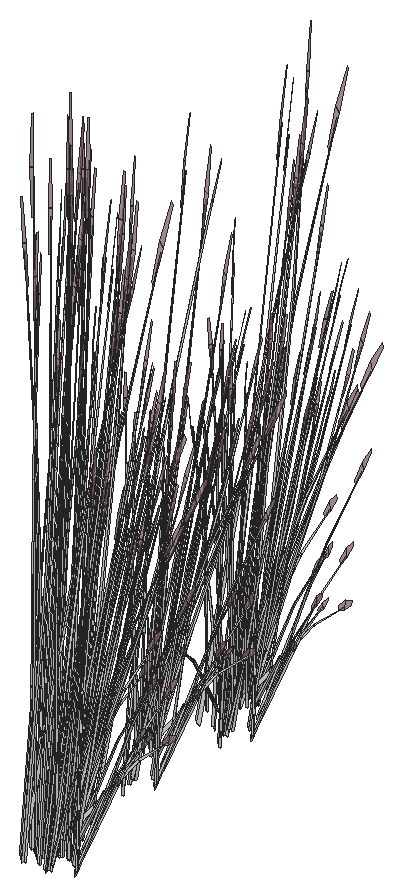
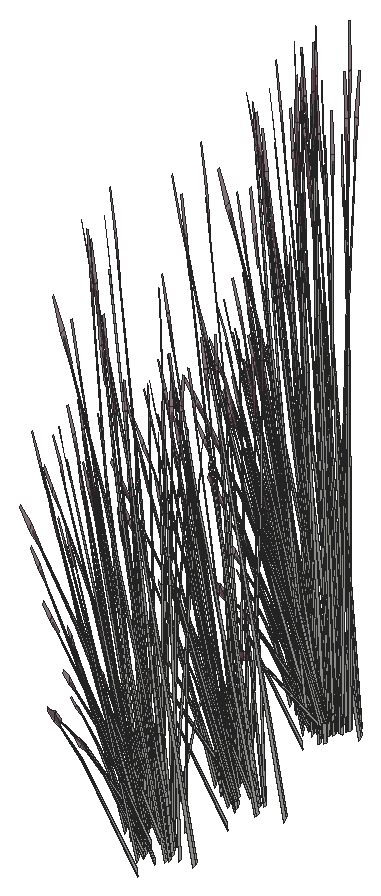
# SketchUp Ruby script. Lengths in inches.
U = 1.inch
M = Sketchup.active_model
def pt(a) = Geom::Point3d.new(a.map { |v| v * U })
def face(e, loops, mat)
  f = e.add_face(loops[0].map { |a| pt(a) })
  loops[1..].each { |l| e.add_face(l.map { |a| pt(a) }).erase! }
  f.material = f.back_material = mat if mat
  f
end
# faces: each face lists its corners as indices into pts; further lists are holes
def faces(e, pts, list, mat = nil) = list.each { |f| face(e, (f[0].is_a?(Array) ? f : [f]).map { |l| l.map { |i| pts[i] } }, mat) }
# xy, xz, yz: faces in a plane at the given z, y or x. An outline is a flat list of corners, or four numbers for a rectangle; further outlines are holes
def ring(l) = l.size == 4 ? [[l[0], l[1]], [l[2], l[1]], [l[2], l[3]], [l[0], l[3]]] : l.each_slice(2).to_a
def flat(e, list, mat, &to3) = list.each { |f| face(e, (f[0].is_a?(Array) ? f : [f]).map { |l| ring(l).map { |u, v| to3.(u, v) } }, mat) }
def xy(e, z, list, mat = nil) = flat(e, list, mat) { |x, y| [x, y, z] }
def xz(e, y, list, mat = nil) = flat(e, list, mat) { |x, z| [x, y, z] }
def yz(e, x, list, mat = nil) = flat(e, list, mat) { |y, z| [x, y, z] }
def lines(e, pts, list) = list.each { |a, b| e.add_line(pt(pts[a]), pt(pts[b])) }
# prism: a flat outline (further loops are holes) pulled along v
def prism(e, loops, v, mat = nil)
  f = face(e, loops, mat); d = Geom::Vector3d.new(v.map { |x| x * U })
  f.pushpull(f.normal.samedirection?(d) ? d.length : -d.length)
end
def box(e, o, s, mat = nil) = prism(e, [[o, [o[0] + s[0], o[1], o[2]], [o[0] + s[0], o[1] + s[1], o[2]], [o[0], o[1] + s[1], o[2]]]], [0, 0, s[2]], mat)
def at(x, y, z, deg = 0) = Geom::Transformation.translation(pt([x, y, z])) * Geom::Transformation.rotation(ORIGIN, Z_AXIS, deg.degrees)
def axes(o, x, y, z) = Geom::Transformation.new([*x, 0, *y, 0, *z, 0, *pt(o).to_a, 1])
def part(name) = M.definitions.add(name)
# library, detail: a bought-in or finely detailed component or shape, given as its bounding box
def library(name, o, s) = part(name).tap { |d| box(d.entities, o, s) }
def detail(e, o, s) = box(e.add_group.entities, o, s)
def put(e, d, t, mat = nil) = e.add_instance(d, t).tap { |i| i.material = mat if mat }
def group(e, t, mat = nil) = e.add_group.tap { |g| g.transformation = t; g.material = mat if mat }.entities
root = M.entities
M.materials.add("LightPink_Translucent").color = [144, 107, 117]
M.materials["LightPink_Translucent"].alpha = 0.75
c1 = part("blade")
p = [[2.15,0.21,22],[0,0.17,0],[0.09,0.45,0],[2.18,0.31,22],[2.29,0.31,22],[0.38,0.45,0],
  [2.48,0.24,33],[2.49,0.24,33],[2.48,0.22,33]]
faces(c1.entities,p,[[0,1,2,3],[4,5,2,3],[6,3,4,7],[8,0,3,6]])
c2 = part("seeds")
p = [[0.3,-0.1,1.38],[-0.01,-0.03,1.59],[-0.01,-0.03,0.03],[0.14,-0.07,-0.07],[0.29,-0.03,3],[0.15,0.01,3.11]]
faces(c2.entities,p,[[0,1,2,3],[1,0,4,5]],"LightPink_Translucent")
c3 = part("blade with seeds")
put(c3.entities,c1,at(0,0,0))
put(c3.entities,c2,axes([2.4,0.25,30.99],[1.5799,-0.05474,1.17369],[-0.12525,1.92788,0.29478],[-0.07173,-0.02425,1.56792]))
put(root,c3,axes([408.35,394.05,-9.42],[-0.17034,0.27669,1.06958],[-0.14642,-0.37174,0.78586],[0.14069,-0.09315,0.23558]))
put(root,c3,axes([408.1,395.09,-7.78],[0.44516,-0.07768,-0.32977],[0.11755,0.44407,0.42575],[0.12757,-0.11927,0.81462]))
put(root,c3,axes([405.49,395.5,-9.52],[-0.05959,-0.62022,-0.27094],[0.62068,-0.0375,-0.46562],[0.1093,-0.08261,1.4872]))
put(root,c3,axes([407.74,395.36,-7.3],[-0.44516,0.07768,0.32977],[-0.11755,-0.44407,-0.42575],[0.12757,-0.11927,0.81462]))
put(root,c3,axes([405.41,394.125,-10.11],[0.47712,0.13449,-0.28847],[-0.12013,0.47362,0.28847],[0.09619,-0.05462,1.29413]))
put(root,c3,axes([408.14,395.29,-7.6],[0.35109,0.22859,0.05988],[-0.2044,0.32553,0.47138],[0.11256,-0.10524,0.71878]))
put(root,c3,axes([408.05,395.1875,-7.59],[0.12683,0.50025,0.447],[-0.49754,0.08682,0.36857],[0.14663,-0.11765,0.92496]))
put(root,c3,axes([409.39,395.79,-7.61],[0.07097,-0.08279,1.62908],[-0.09083,-0.50786,-0.25764],[0.17806,-0.09629,0.13065]))
put(root,c3,axes([405.57,395.98,-9.73],[0.57623,0.26344,0.22409],[-0.27732,0.5474,0.46562],[0,-0.12618,1.49497]))
put(root,c3,axes([405.39,395.62,-9.47],[-0.55535,0.03355,0.41661],[-0.05022,-0.55698,-0.2005],[0.09942,-0.05645,1.33761]))
put(root,c3,axes([407.99,396.57,-7.3125],[-0.25732,-0.49218,-0.11324],[0.45669,-0.24187,-0.62851],[0.19245,-0.06494,0.95501]))
put(root,c3,axes([407.97,396.14,-7.64],[0.13855,-0.49442,-0.47583],[0.47502,0.16947,-0.36857],[0.19125,-0.04534,0.91046]))
put(root,c3,axes([407.22,394.13,-9.79],[0.31974,-0.54466,0],[0.53494,0.30375,-0.48057],[0.12184,0.06918,1.52448]))
put(root,c3,axes([408.48,396.28,-10.15],[-0.32938,0.06523,1.31842],[-0.05243,-0.51922,0.07547],[0.2307,-0.07859,0.75023]))
put(root,c3,axes([409.08,395.82,-9.89],[-0.31706,-0.34757,-0.06041],[0.34725,-0.31847,-0.27392],[0.09839,-0.02242,0.90349]))
put(root,c3,axes([406.17,395.87,-9.95],[0,-0.62892,0],[0.63949,0,0],[0,0,1.6711]))
put(root,c3,axes([406.94,394.41,-9.69],[-0.47863,-0.27177,0.46235],[0.28609,-0.48733,0],[0.10901,0.0619,1.46668]))
put(root,c3,axes([407.88,396.32,-7.36],[0.44939,-0.24006,-0.66157],[0.25044,0.49415,0.07984],[0.21713,-0.05613,0.93586]))
put(root,c3,axes([405.86,395.47,-9.8],[-0.42403,0.49328,0.42607],[-0.50377,-0.43543,0.16719],[0.10223,-0.04923,1.47927]))
put(root,c3,axes([405.125,394.66,-9.7],[-0.14774,0.54019,0.16428],[-0.54062,-0.15287,0.32672],[0.09339,-0.00263,1.49371]))
put(root,c3,axes([407.8125,396.42,-7.3],[-0.42502,-0.15163,0.32977],[0.12396,-0.44238,-0.42575],[0.17112,-0.04056,0.81462]))
put(root,c3,axes([404.9,395.1,-10.52],[-0.50338,0.21762,1.20058],[-0.16022,-0.62439,0.4665],[0.30911,0.01039,1.36553]))
put(root,c3,axes([406.26,395.26,-9.5625],[0.09866,-0.48509,0.13483],[0.48202,0.0842,-0.38503],[0.08772,0.04981,1.18024]))
put(root,c3,axes([408.83,395.94,-10.61],[-0.02673,-0.08252,1.6421],[0.18538,-0.48271,-0.25086],[0.187,-0.00694,0.2797]))
put(root,c3,axes([406.05,395.39,-9.47],[-0.30722,-0.45622,0.41661],[0.46535,-0.32126,-0.2005],[0.09942,0.05645,1.33761]))
put(root,c3,axes([406.21,395.42,-9.52],[0.51635,-0.36087,-0.27094],[0.34336,0.5099,-0.46562],[0.1274,0.05178,1.4872]))
put(root,c3,axes([408.26,396.37,-7.78],[0.42502,0.15163,-0.32977],[-0.12396,0.44238,0.42575],[0.17112,-0.04056,0.81462]))
put(root,c3,axes([407.51,394.46,-10.12],[0.47863,0.27177,-0.46235],[-0.28609,0.48733,0],[0.10901,0.0619,1.46668]))
put(root,c3,axes([406.6,396.01,-9.95],[0.57217,0,0],[0,0.56272,0],[0,0,1.66132]))
put(root,c3,axes([406.76,394.6875,-9.7],[-0.54955,0.14427,0.16428],[-0.1357,-0.53689,0.32672],[0.04901,0.07823,1.49371]))
put(root,c3,axes([407.1,395.82,-8.39],[-0.21212,0.01231,1.59586],[0.14072,-0.53355,0.12904],[0.3023,0.033,0.68222]))
put(root,c3,axes([407.375,394.66,-10.11],[0.12013,0.47362,-0.28847],[-0.47712,0.13449,0.28847],[0.09619,0.05462,1.29413]))
put(root,c3,axes([408.2,396.56,-7.6],[0.18783,0.37061,0.05988],[-0.34252,0.1814,0.47138],[0.15099,-0.03579,0.71878]))
put(root,c3,axes([406.42,395.72,-9.78],[-0.64638,-0.11452,0.45814],[0.13155,-0.64678,0.17978],[0.09446,0.06245,1.59061]))
put(root,c3,axes([408.16,396.42,-7.59],[-0.14449,0.4956,0.447],[-0.47502,-0.16947,0.36857],[0.1868,-0.02978,0.92496]))
put(root,c3,axes([406.52,397.25,-9.97],[0.53691,-0.18442,-0.17877],[0.18866,0.53125,0.00007],[0.05927,-0.02038,1.61933]))
put(root,c3,axes([406.59,396.25,-9.9375],[0.35699,0.35109,0],[-0.35699,0.35109,0],[0,0,1.57621]))
put(root,c3,axes([407.55,396.1,-9.7],[-0.40181,-0.39593,0.16428],[0.40492,-0.38402,0.32672],[-0.04438,0.08086,1.49371]))
put(root,c3,axes([406.81,395.5,-10.08],[0.53199,0.08911,-0.58063],[-0.11226,0.54969,-0.15239],[0.15876,0.06661,1.28164]))
put(root,c3,axes([409.16,396.46,-9.42],[-0.31598,0.08973,1.06958],[0.14873,-0.37085,0.78586],[0.16763,0.02538,0.23558]))
put(root,c3,axes([406.58,395.84,-9.47],[0.24813,-0.48978,0.41661],[0.51557,0.23571,-0.2005],[0,0.1129,1.33761]))
put(root,c3,axes([409.01,398.03,-7.62],[-0.04624,-0.04758,1.65179],[0.10116,-0.51007,-0.15608],[0.18215,-0.03259,0.29231]))
put(root,c3,axes([406.49,396.12,-9.87],[0,0.62861,-0.05249],[-0.63949,0,0],[0,0.01975,1.67027]))
put(root,c3,axes([406.53,395.67,-9.94],[0.30722,0.45622,-0.41661],[-0.46535,0.32126,0.2005],[0.09942,0.05645,1.33761]))
put(root,c3,axes([408.61,397.6,-8.34],[-0.09788,-0.45691,-0.03251],[0.46264,-0.10504,-0.14742],[0.09661,0.02897,0.48626]))
put(root,c3,axes([407.41,397.59,-7.3125],[0.02738,-0.55277,-0.11324],[0.51847,0.01511,-0.62851],[0.19968,0.0384,0.95501]))
put(root,c3,axes([407.89,396.11,-9.69],[0,-0.54355,0.46235],[0.57217,0,0],[0,0.1238,1.46668]))
put(root,c3,axes([406.8,395.95,-9.5625],[0.47648,-0.15851,0.13483],[0.16686,0.45265,-0.38503],[0,0.09962,1.18024]))
put(root,c3,axes([407.33,397.37,-7.3],[-0.29098,-0.34031,0.32977],[0.33226,-0.32215,-0.42575],[0.16881,0.04902,0.81462]))
put(root,c3,axes([408.57,397.05,-9.59],[-0.12317,-0.13368,1.33163],[0.16025,-0.44223,-0.28638],[0.24919,0.05991,0.56934]))
put(root,c3,axes([406.37,397.54,-9.95],[0.51557,0.24403,0],[-0.24813,0.50705,0],[0,0,1.62917]))
put(root,c3,axes([407.86,397.26,-7.61],[0.10971,-0.00919,1.62908],[0.30091,-0.42228,-0.25764],[0.19514,0.05574,0.13065]))
put(root,c3,axes([407.4375,397.32,-7.36],[0.51122,0.01309,-0.66157],[-0.03434,0.5511,0.07984],[0.21658,0.05816,0.93586]))
put(root,c3,axes([406.18,397.34,-9.87],[0.22235,0.62444,-0.05599],[-0.63531,0.21881,0],[0.00776,0.02181,1.60327]))
put(root,c3,axes([408.27,396.2,-9.79],[0.63949,0,0],[0,0.60749,-0.48057],[0,0.13836,1.52448]))
put(root,c3,axes([408.02,396.52,-9.95],[-0.63917,-0.00435,-0.04634],[0,-0.60749,0.46507],[-0.02009,0.13829,1.47457]))
put(root,c3,axes([406.63,395.99,-9.52],[0.57594,0.25935,-0.27094],[-0.27732,0.5474,-0.46562],[0.0181,0.1344,1.4872]))
put(root,c3,axes([407.75,397.55,-7.78],[0.29098,0.34031,-0.32977],[-0.33226,0.32215,0.42575],[0.16881,0.04902,0.81462]))
put(root,c3,axes([407.89,396.6,-10.11],[-0.35699,0.33913,-0.28847],[-0.35699,-0.33913,0.28847],[0,0.10923,1.29413]))
put(root,c3,axes([407.6,397.68,-7.6],[-0.02575,0.41332,0.05988],[-0.38885,-0.01133,0.47138],[0.14895,0.04325,0.71878]))
put(root,c3,axes([407.63,397.55,-7.59],[-0.37709,0.35815,0.447],[-0.32522,-0.38035,0.36857],[0.17692,0.06607,0.92496]))
put(root,c3,axes([406.43,397.96,-7.3],[-0.07899,-0.43781,0.32977],[0.45153,-0.11561,-0.42575],[0.12128,0.12546,0.81462]))
put(root,c3,axes([408.13,396.62,-10.12],[0,0.54355,-0.46235],[-0.57217,0,0],[0,0.1238,1.46668]))
put(root,c3,axes([406.7,396.68,-8.39],[-0.18996,-0.09365,1.59586],[0.39312,-0.39287,0.12904],[0.24502,0.17723,0.68222]))
put(root,c3,axes([406.74,395.44,-7.83],[-0.44191,-0.28242,1.28769],[0.46662,-0.43971,0.5556],[0.14258,0.26499,1.24467]))
put(root,c3,axes([407.4,397.74,-9.42],[-0.28795,-0.15629,1.06958],[0.37181,-0.1588,0.78586],[0.10029,0.13452,0.23558]))
put(root,c3,axes([406.39,398.19,-7.3125],[0.30474,-0.46525,-0.11324],[0.44133,0.26804,-0.62851],[0.15341,0.13145,0.95501]))
put(root,c3,axes([405.99,398.58,-7.62],[0.00151,-0.06581,1.65179],[0.43826,-0.29033,-0.15608],[0.15223,0.10363,0.29231]))
put(root,c3,axes([407.48,398.32,-10.61],[0.03726,-0.07847,1.6421],[0.46909,-0.23111,-0.25086],[0.14221,0.11962,0.2797]))
put(root,c3,axes([406.87,396.54,-10.05],[0.18752,0.49766,-0.6445],[-0.54017,0.17923,-0.16915],[0.02073,0.16852,1.42262]))
put(root,c3,axes([406.75,397.96,-7.64],[0.50465,-0.12921,-0.47583],[0.08828,0.48932,-0.36857],[0.13555,0.14022,0.91046]))
put(root,c3,axes([405.35,398.03,-7.3],[0.15418,-0.41799,0.32977],[0.44981,0.12192,-0.42575],[0.04124,0.16829,0.81462]))
put(root,c3,axes([407.45,398.46,-9.52],[-0.32795,-0.01705,0.97832],[0.21658,-0.36206,0.54015],[0.12956,0.12863,0.76741]))
put(root,c3,axes([406.5,398.36,-7.6],[-0.23243,0.34529,0.05988],[-0.331,-0.20103,0.47138],[0.10701,0.1107,0.71878]))
put(root,c3,axes([405.96,399.52,-6.74],[0.35341,-0.31182,-0.06041],[0.32382,0.34152,-0.27392],[0.0228,0.09677,0.90349]))
put(root,c3,axes([406.6,398.26,-7.59],[-0.50866,0.12474,0.447],[-0.08828,-0.48932,0.36857],[0.11963,0.14421,0.92496]))
put(root,c3,axes([406.38,397.58,-9.59],[0.00902,-0.18018,1.33163],[0.43127,-0.20126,-0.28638],[0.13313,0.21566,0.56934]))
put(root,c3,axes([405.2,398.21,-7.3125],[0.50045,-0.25306,-0.11324],[0.24593,0.44915,-0.62851],[0.06603,0.18927,0.95501]))
put(root,c3,axes([405.63,398.1875,-7.64],[0.50273,0.13626,-0.47583],[-0.17232,0.46717,-0.36857],[0.0461,0.18809,0.91046]))
put(root,c3,axes([405.92,397.22,-8.39],[-0.1169,-0.17452,1.59586],[0.54019,-0.14692,0.12904],[0.12209,0.27397,0.68222]))
put(root,c3,axes([405.45,398.1,-7.36],[0.24409,0.44196,-0.66157],[-0.50245,0.2463,0.07984],[0.05708,0.21354,0.93586]))
put(root,c3,axes([405.08,399.21,-7.61],[0.06483,0.08753,1.62908],[0.52315,0.03439,-0.25764],[0.05261,0.19303,0.13065]))
put(root,c3,axes([404.36,407.02,-10.61],[-0.07655,-0.04282,1.6421],[-0.19662,-0.47839,-0.25086],[0.13264,-0.12982,0.2797]))
put(root,c3,axes([404.36,408.37,-7.36],[0.26714,-0.42887,-0.66157],[0.46811,0.30479,0.07984],[0.1595,-0.15539,0.93586]))
put(root,c3,axes([404.35,408.17,-7.64],[-0.13138,-0.49631,-0.47583],[0.49754,-0.08682,-0.36857],[0.14258,-0.13331,0.91046]))
put(root,c3,axes([404.58,408.52,-7.3125],[-0.47307,-0.29971,-0.11324],[0.27254,-0.43404,-0.62851],[0.13365,-0.15087,0.95501]))
put(root,c3,axes([404.75,407.98,-9.59],[-0.1827,-0.0161,1.33163],[-0.18717,-0.43188,-0.28638],[0.22444,-0.12218,0.56934]))
put(root,c3,axes([405.75,408.39,-7.62],[-0.0668,-0.00413,1.65179],[-0.27738,-0.44233,-0.15608],[0.11139,-0.14544,0.29231]))
put(root,c3,axes([404.96,407.18,-9.42],[-0.17034,0.27669,1.06958],[-0.14642,-0.37174,0.78586],[0.14069,-0.09315,0.23558]))
put(root,c3,axes([404.71,408.22,-7.78],[0.44516,-0.07768,-0.32977],[0.11755,0.44407,0.42575],[0.12757,-0.11927,0.81462]))
put(root,c3,axes([404.75,408.41,-7.6],[0.35109,0.22859,0.05988],[-0.2044,0.32553,0.47138],[0.11256,-0.10524,0.71878]))
put(root,c3,axes([404.66,408.32,-7.59],[0.12683,0.50025,0.447],[-0.49754,0.08682,0.36857],[0.14663,-0.11765,0.92496]))
put(root,c3,axes([406,408.92,-7.61],[0.07097,-0.08279,1.62908],[-0.09083,-0.50786,-0.25764],[0.17806,-0.09629,0.13065]))
put(root,c3,axes([404.6,409.69,-7.3125],[-0.25732,-0.49218,-0.11324],[0.45669,-0.24187,-0.62851],[0.19245,-0.06494,0.95501]))
put(root,c3,axes([404.58,409.27,-7.64],[0.13855,-0.49442,-0.47583],[0.47502,0.16947,-0.36857],[0.19125,-0.04534,0.91046]))
put(root,c3,axes([403.83,407.26,-9.79],[0.31974,-0.54466,0],[0.53494,0.30375,-0.48057],[0.12184,0.06918,1.52448]))
put(root,c3,axes([405.09,409.41,-10.15],[-0.32938,0.06523,1.31842],[-0.05243,-0.51922,0.07547],[0.2307,-0.07859,0.75023]))
put(root,c3,axes([405.69,408.95,-9.89],[-0.31706,-0.34757,-0.06041],[0.34725,-0.31847,-0.27392],[0.09839,-0.02242,0.90349]))
put(root,c3,axes([404.49,409.45,-7.36],[0.44939,-0.24006,-0.66157],[0.25044,0.49415,0.07984],[0.21713,-0.05613,0.93586]))
put(root,c3,axes([404.42,409.55,-7.3],[-0.42502,-0.15163,0.32977],[0.12396,-0.44238,-0.42575],[0.17112,-0.04056,0.81462]))
put(root,c3,axes([401.51,408.22,-10.52],[-0.50338,0.21762,1.20058],[-0.16022,-0.62439,0.4665],[0.30911,0.01039,1.36553]))
put(root,c3,axes([405.44,409.07,-10.61],[-0.02673,-0.08252,1.6421],[0.18538,-0.48271,-0.25086],[0.187,-0.00694,0.2797]))
put(root,c3,axes([404.87,409.5,-7.78],[0.42502,0.15163,-0.32977],[-0.12396,0.44238,0.42575],[0.17112,-0.04056,0.81462]))
put(root,c3,axes([404.12,407.59,-10.12],[0.47863,0.27177,-0.46235],[-0.28609,0.48733,0],[0.10901,0.0619,1.46668]))
put(root,c3,axes([403.71,408.95,-8.39],[-0.21212,0.01231,1.59586],[0.14072,-0.53355,0.12904],[0.3023,0.033,0.68222]))
put(root,c3,axes([404.81,409.68,-7.6],[0.18783,0.37061,0.05988],[-0.34252,0.1814,0.47138],[0.15099,-0.03579,0.71878]))
put(root,c3,axes([404.77,409.55,-7.59],[-0.14449,0.4956,0.447],[-0.47502,-0.16947,0.36857],[0.1868,-0.02978,0.92496]))
put(root,c3,axes([403.42,408.63,-10.08],[0.53199,0.08911,-0.58063],[-0.11226,0.54969,-0.15239],[0.15876,0.06661,1.28164]))
put(root,c3,axes([405.77,409.59,-9.42],[-0.31598,0.08973,1.06958],[0.14873,-0.37085,0.78586],[0.16763,0.02538,0.23558]))
put(root,c3,axes([405.625,411.16,-7.62],[-0.04624,-0.04758,1.65179],[0.10116,-0.51007,-0.15608],[0.18215,-0.03259,0.29231]))
put(root,c3,axes([405.22,410.73,-8.34],[-0.09788,-0.45691,-0.03251],[0.46264,-0.10504,-0.14742],[0.09661,0.02897,0.48626]))
put(root,c3,axes([404.02,410.72,-7.3125],[0.02738,-0.55277,-0.11324],[0.51847,0.01511,-0.62851],[0.19968,0.0384,0.95501]))
put(root,c3,axes([403.94,410.5,-7.3],[-0.29098,-0.34031,0.32977],[0.33226,-0.32215,-0.42575],[0.16881,0.04902,0.81462]))
put(root,c3,axes([405.18,410.18,-9.59],[-0.12317,-0.13368,1.33163],[0.16025,-0.44223,-0.28638],[0.24919,0.05991,0.56934]))
put(root,c3,axes([404.47,410.39,-7.61],[0.10971,-0.00919,1.62908],[0.30091,-0.42228,-0.25764],[0.19514,0.05574,0.13065]))
put(root,c3,axes([404.05,410.45,-7.36],[0.51122,0.01309,-0.66157],[-0.03434,0.5511,0.07984],[0.21658,0.05816,0.93586]))
put(root,c3,axes([404.36,410.68,-7.78],[0.29098,0.34031,-0.32977],[-0.33226,0.32215,0.42575],[0.16881,0.04902,0.81462]))
put(root,c3,axes([404.21,410.81,-7.6],[-0.02575,0.41332,0.05988],[-0.38885,-0.01133,0.47138],[0.14895,0.04325,0.71878]))
put(root,c3,axes([404.24,410.68,-7.59],[-0.37709,0.35815,0.447],[-0.32522,-0.38035,0.36857],[0.17692,0.06607,0.92496]))
put(root,c3,axes([405.43,416.3125,-7.61],[-0.00494,-0.10818,1.62908],[-0.41695,-0.31265,-0.25764],[0.06446,-0.18952,0.13065]))
put(root,c3,axes([404.02,416.84,-8.39],[-0.09522,0.18683,1.59586],[-0.39947,-0.38663,0.12904],[0.18021,-0.24097,0.68222]))
put(root,c3,axes([403.31,409.81,-8.39],[-0.18996,-0.09365,1.59586],[0.39312,-0.39287,0.12904],[0.24502,0.17723,0.68222]))
put(root,c3,axes([403,411.32,-7.3125],[0.30474,-0.46525,-0.11324],[0.44133,0.26804,-0.62851],[0.15341,0.13145,0.95501]))
put(root,c3,axes([404.88,416.79,-7.78],[0.34603,-0.28618,-0.32977],[0.32756,0.32677,0.42575],[0.04984,-0.16603,0.81462]))
put(root,c3,axes([404.09,411.45,-10.61],[0.03726,-0.07847,1.6421],[0.46909,-0.23111,-0.25086],[0.14221,0.11962,0.2797]))
put(root,c3,axes([403.36,411.09,-7.64],[0.50465,-0.12921,-0.47583],[0.08828,0.48932,-0.36857],[0.13555,0.14022,0.91046]))
put(root,c3,axes([405.3125,416.62,-10.61],[-0.07655,-0.04282,1.6421],[-0.19662,-0.47839,-0.25086],[0.13264,-0.12982,0.2797]))
put(root,c3,axes([404.88,416.91,-7.59],[0.36417,0.37086,0.447],[-0.38674,0.31985,0.36857],[0.06718,-0.174,0.92496]))
put(root,c3,axes([405.01,416.94,-7.6],[0.42027,0.02533,0.05988],[-0.01152,0.38243,0.47138],[0.04398,-0.14649,0.71878]))
put(root,c3,axes([405.3125,417.97,-7.36],[0.26714,-0.42887,-0.66157],[0.46811,0.30479,0.07984],[0.1595,-0.15539,0.93586]))
put(root,c3,axes([405.3,417.77,-7.64],[-0.13138,-0.49631,-0.47583],[0.49754,-0.08682,-0.36857],[0.14258,-0.13331,0.91046]))
put(root,c3,axes([405.53,418.125,-7.3125],[-0.47307,-0.29971,-0.11324],[0.27254,-0.43404,-0.62851],[0.13365,-0.15087,0.95501]))
put(root,c3,axes([405.7,417.58,-9.59],[-0.1827,-0.0161,1.33163],[-0.18717,-0.43188,-0.28638],[0.22444,-0.12218,0.56934]))
put(root,c3,axes([406.7,418,-7.62],[-0.0668,-0.00413,1.65179],[-0.27738,-0.44233,-0.15608],[0.11139,-0.14544,0.29231]))
put(root,c3,axes([403.42,417.75,-10.08],[0.34446,-0.40855,-0.58063],[0.42791,0.37046,-0.15239],[0.13803,-0.10191,1.28164]))
put(root,c3,axes([405.91,416.78,-9.42],[-0.17034,0.27669,1.06958],[-0.14642,-0.37174,0.78586],[0.14069,-0.09315,0.23558]))
put(root,c3,axes([405.66,417.82,-7.78],[0.44516,-0.07768,-0.32977],[0.11755,0.44407,0.42575],[0.12757,-0.11927,0.81462]))
put(root,c3,axes([405.3,418.09,-7.3],[-0.44516,0.07768,0.32977],[-0.11755,-0.44407,-0.42575],[0.12757,-0.11927,0.81462]))
put(root,c3,axes([405.7,418.02,-7.6],[0.35109,0.22859,0.05988],[-0.2044,0.32553,0.47138],[0.11256,-0.10524,0.71878]))
put(root,c3,axes([405.61,417.92,-7.59],[0.12683,0.50025,0.447],[-0.49754,0.08682,0.36857],[0.14663,-0.11765,0.92496]))
put(root,c3,axes([406.95,418.52,-7.61],[0.07097,-0.08279,1.62908],[-0.09083,-0.50786,-0.25764],[0.17806,-0.09629,0.13065]))
put(root,c3,axes([405.55,419.3,-7.3125],[-0.25732,-0.49218,-0.11324],[0.45669,-0.24187,-0.62851],[0.19245,-0.06494,0.95501]))
put(root,c3,axes([405.53,418.875,-7.64],[0.13855,-0.49442,-0.47583],[0.47502,0.16947,-0.36857],[0.19125,-0.04534,0.91046]))
put(root,c3,axes([404.78,416.86,-9.79],[0.31974,-0.54466,0],[0.53494,0.30375,-0.48057],[0.12184,0.06918,1.52448]))
put(root,c3,axes([406.04,419.01,-10.15],[-0.32938,0.06523,1.31842],[-0.05243,-0.51922,0.07547],[0.2307,-0.07859,0.75023]))
put(root,c3,axes([406.64,418.55,-9.89],[-0.31706,-0.34757,-0.06041],[0.34725,-0.31847,-0.27392],[0.09839,-0.02242,0.90349]))
put(root,c3,axes([405.4375,419.05,-7.36],[0.44939,-0.24006,-0.66157],[0.25044,0.49415,0.07984],[0.21713,-0.05613,0.93586]))
put(root,c3,axes([405.37,419.15,-7.3],[-0.42502,-0.15163,0.32977],[0.12396,-0.44238,-0.42575],[0.17112,-0.04056,0.81462]))
put(root,c3,axes([402.46,417.83,-10.52],[-0.50338,0.21762,1.20058],[-0.16022,-0.62439,0.4665],[0.30911,0.01039,1.36553]))
put(root,c3,axes([406.4,418.67,-10.61],[-0.02673,-0.08252,1.6421],[0.18538,-0.48271,-0.25086],[0.187,-0.00694,0.2797]))
put(root,c3,axes([403.77,418.15,-9.52],[0.51635,-0.36087,-0.27094],[0.34336,0.5099,-0.46562],[0.1274,0.05178,1.4872]))
put(root,c3,axes([405.82,419.1,-7.78],[0.42502,0.15163,-0.32977],[-0.12396,0.44238,0.42575],[0.17112,-0.04056,0.81462]))
put(root,c3,axes([405.07,417.1875,-10.12],[0.47863,0.27177,-0.46235],[-0.28609,0.48733,0],[0.10901,0.0619,1.46668]))
put(root,c3,axes([404.66,418.55,-8.39],[-0.21212,0.01231,1.59586],[0.14072,-0.53355,0.12904],[0.3023,0.033,0.68222]))
put(root,c3,axes([404.9375,417.39,-10.11],[0.12013,0.47362,-0.28847],[-0.47712,0.13449,0.28847],[0.09619,0.05462,1.29413]))
put(root,c3,axes([405.76,419.28,-7.6],[0.18783,0.37061,0.05988],[-0.34252,0.1814,0.47138],[0.15099,-0.03579,0.71878]))
put(root,c3,axes([405.72,419.15,-7.59],[-0.14449,0.4956,0.447],[-0.47502,-0.16947,0.36857],[0.1868,-0.02978,0.92496]))
put(root,c3,axes([404.37,418.23,-10.08],[0.53199,0.08911,-0.58063],[-0.11226,0.54969,-0.15239],[0.15876,0.06661,1.28164]))
put(root,c3,axes([406.72,419.1875,-9.42],[-0.31598,0.08973,1.06958],[0.14873,-0.37085,0.78586],[0.16763,0.02538,0.23558]))
put(root,c3,axes([406.57,420.76,-7.62],[-0.04624,-0.04758,1.65179],[0.10116,-0.51007,-0.15608],[0.18215,-0.03259,0.29231]))
put(root,c3,axes([404.09,418.4,-9.94],[0.30722,0.45622,-0.41661],[-0.46535,0.32126,0.2005],[0.09942,0.05645,1.33761]))
put(root,c3,axes([406.17,420.33,-8.34],[-0.09788,-0.45691,-0.03251],[0.46264,-0.10504,-0.14742],[0.09661,0.02897,0.48626]))
put(root,c3,axes([404.97,420.32,-7.3125],[0.02738,-0.55277,-0.11324],[0.51847,0.01511,-0.62851],[0.19968,0.0384,0.95501]))
put(root,c3,axes([404.89,420.1,-7.3],[-0.29098,-0.34031,0.32977],[0.33226,-0.32215,-0.42575],[0.16881,0.04902,0.81462]))
put(root,c3,axes([406.13,419.78,-9.59],[-0.12317,-0.13368,1.33163],[0.16025,-0.44223,-0.28638],[0.24919,0.05991,0.56934]))
put(root,c3,axes([405.42,419.99,-7.61],[0.10971,-0.00919,1.62908],[0.30091,-0.42228,-0.25764],[0.19514,0.05574,0.13065]))
put(root,c3,axes([405,420.05,-7.36],[0.51122,0.01309,-0.66157],[-0.03434,0.5511,0.07984],[0.21658,0.05816,0.93586]))
put(root,c3,axes([405.83,418.93,-9.79],[0.63949,0,0],[0,0.60749,-0.48057],[0,0.13836,1.52448]))
put(root,c3,axes([405.31,420.28,-7.78],[0.29098,0.34031,-0.32977],[-0.33226,0.32215,0.42575],[0.16881,0.04902,0.81462]))
put(root,c3,axes([405.16,420.41,-7.6],[-0.02575,0.41332,0.05988],[-0.38885,-0.01133,0.47138],[0.14895,0.04325,0.71878]))
put(root,c3,axes([405.19,420.28,-7.59],[-0.37709,0.35815,0.447],[-0.32522,-0.38035,0.36857],[0.17692,0.06607,0.92496]))
put(root,c3,axes([404.26,419.41,-8.39],[-0.18996,-0.09365,1.59586],[0.39312,-0.39287,0.12904],[0.24502,0.17723,0.68222]))
put(root,c3,axes([404.3,418.17,-7.83],[-0.44191,-0.28242,1.28769],[0.46662,-0.43971,0.5556],[0.14258,0.26499,1.24467]))
put(root,c3,axes([404.96,420.47,-9.42],[-0.28795,-0.15629,1.06958],[0.37181,-0.1588,0.78586],[0.10029,0.13452,0.23558]))
put(root,c3,axes([403.95,420.92,-7.3125],[0.30474,-0.46525,-0.11324],[0.44133,0.26804,-0.62851],[0.15341,0.13145,0.95501]))
put(root,c3,axes([403.55,421.31,-7.62],[0.00151,-0.06581,1.65179],[0.43826,-0.29033,-0.15608],[0.15223,0.10363,0.29231]))
put(root,c3,axes([405.04,421.05,-10.61],[0.03726,-0.07847,1.6421],[0.46909,-0.23111,-0.25086],[0.14221,0.11962,0.2797]))
put(root,c3,axes([404.3125,420.6875,-7.64],[0.50465,-0.12921,-0.47583],[0.08828,0.48932,-0.36857],[0.13555,0.14022,0.91046]))
put(root,c3,axes([405.01,421.19,-9.52],[-0.32795,-0.01705,0.97832],[0.21658,-0.36206,0.54015],[0.12956,0.12863,0.76741]))
put(root,c3,axes([403.9375,420.31,-9.59],[0.00902,-0.18018,1.33163],[0.43127,-0.20126,-0.28638],[0.13313,0.21566,0.56934]))
